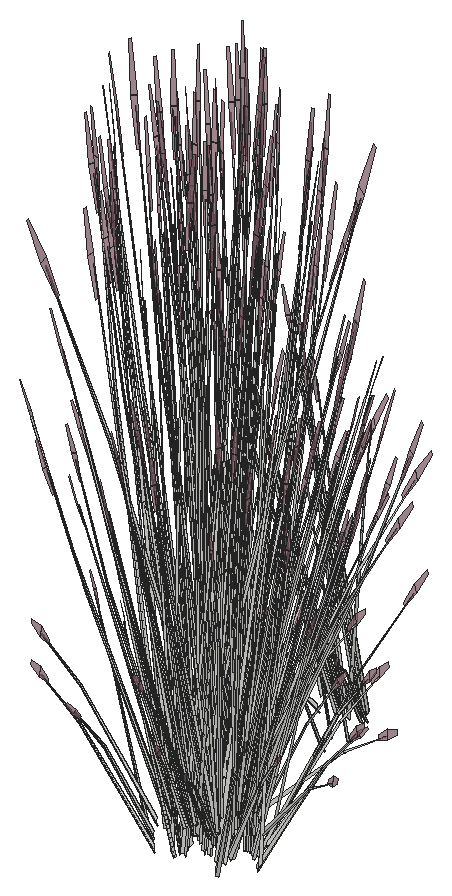
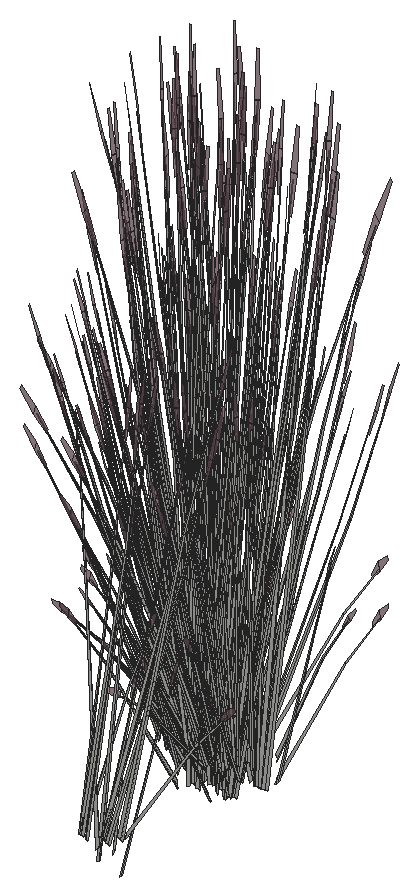
# SketchUp Ruby script. Lengths in inches.
U = 1.inch
M = Sketchup.active_model
def pt(a) = Geom::Point3d.new(a.map { |v| v * U })
def face(e, loops, mat)
  f = e.add_face(loops[0].map { |a| pt(a) })
  loops[1..].each { |l| e.add_face(l.map { |a| pt(a) }).erase! }
  f.material = f.back_material = mat if mat
  f
end
# faces: each face lists its corners as indices into pts; further lists are holes
def faces(e, pts, list, mat = nil) = list.each { |f| face(e, (f[0].is_a?(Array) ? f : [f]).map { |l| l.map { |i| pts[i] } }, mat) }
# xy, xz, yz: faces in a plane at the given z, y or x. An outline is a flat list of corners, or four numbers for a rectangle; further outlines are holes
def ring(l) = l.size == 4 ? [[l[0], l[1]], [l[2], l[1]], [l[2], l[3]], [l[0], l[3]]] : l.each_slice(2).to_a
def flat(e, list, mat, &to3) = list.each { |f| face(e, (f[0].is_a?(Array) ? f : [f]).map { |l| ring(l).map { |u, v| to3.(u, v) } }, mat) }
def xy(e, z, list, mat = nil) = flat(e, list, mat) { |x, y| [x, y, z] }
def xz(e, y, list, mat = nil) = flat(e, list, mat) { |x, z| [x, y, z] }
def yz(e, x, list, mat = nil) = flat(e, list, mat) { |y, z| [x, y, z] }
def lines(e, pts, list) = list.each { |a, b| e.add_line(pt(pts[a]), pt(pts[b])) }
# prism: a flat outline (further loops are holes) pulled along v
def prism(e, loops, v, mat = nil)
  f = face(e, loops, mat); d = Geom::Vector3d.new(v.map { |x| x * U })
  f.pushpull(f.normal.samedirection?(d) ? d.length : -d.length)
end
def box(e, o, s, mat = nil) = prism(e, [[o, [o[0] + s[0], o[1], o[2]], [o[0] + s[0], o[1] + s[1], o[2]], [o[0], o[1] + s[1], o[2]]]], [0, 0, s[2]], mat)
def at(x, y, z, deg = 0) = Geom::Transformation.translation(pt([x, y, z])) * Geom::Transformation.rotation(ORIGIN, Z_AXIS, deg.degrees)
def axes(o, x, y, z) = Geom::Transformation.new([*x, 0, *y, 0, *z, 0, *pt(o).to_a, 1])
def part(name) = M.definitions.add(name)
# library, detail: a bought-in or finely detailed component or shape, given as its bounding box
def library(name, o, s) = part(name).tap { |d| box(d.entities, o, s) }
def detail(e, o, s) = box(e.add_group.entities, o, s)
def put(e, d, t, mat = nil) = e.add_instance(d, t).tap { |i| i.material = mat if mat }
def group(e, t, mat = nil) = e.add_group.tap { |g| g.transformation = t; g.material = mat if mat }.entities
root = M.entities
M.materials.add("LightPink_Translucent").color = [144, 107, 117]
M.materials["LightPink_Translucent"].alpha = 0.75
c1 = part("blade")
p = [[2.15,0.21,22],[0,0.17,0],[0.09,0.45,0],[2.18,0.31,22],[2.29,0.31,22],[0.38,0.45,0],
  [2.48,0.24,33],[2.49,0.24,33],[2.48,0.22,33]]
faces(c1.entities,p,[[0,1,2,3],[4,5,2,3],[6,3,4,7],[8,0,3,6]])
c2 = part("seeds")
p = [[0.3,-0.1,1.38],[-0.01,-0.03,1.59],[-0.01,-0.03,0.03],[0.14,-0.07,-0.07],[0.29,-0.03,3],[0.15,0.01,3.11]]
faces(c2.entities,p,[[0,1,2,3],[1,0,4,5]],"LightPink_Translucent")
c3 = part("blade with seeds")
put(c3.entities,c1,at(0,0,0))
put(c3.entities,c2,axes([2.4,0.25,30.99],[1.5799,-0.05474,1.17369],[-0.12525,1.92788,0.29478],[-0.07173,-0.02425,1.56792]))
put(root,c3,axes([512.9,457.95,3.91],[-0.00733,-0.12161,1.74944],[-0.61946,-0.35147,-0.27667],[0.09577,-0.21306,0.14031]))
put(root,c3,axes([510.3,457.92,3.72],[0.22906,-0.4699,-0.35414],[0.66828,0.13705,0.4572],[-0.06128,-0.18919,0.87481]))
put(root,c3,axes([510.8,458.55,3.07],[-0.14147,0.21002,1.71376],[-0.59349,-0.43464,0.13857],[0.26773,-0.27089,0.73262]))
put(root,c3,axes([512.73,457.51,3.9],[-0.07716,0.04667,1.77383],[-0.75601,-0.15746,-0.16761],[-0.02737,-0.20368,0.31391]))
put(root,c3,axes([509.96,458.25,3.875],[-0.7469,-0.15318,-0.51099],[0.25601,-0.52518,-0.3958],[-0.06849,-0.21144,0.97773]))
put(root,c3,axes([510.42,456.93,1.96],[0.09747,0.35631,1.1486],[-0.54071,-0.19735,0.84392],[0.05818,-0.18244,0.25299]))
put(root,c3,axes([511.57,458.64,3.875],[-0.54391,-0.41056,-0.51099],[0.57458,-0.35956,-0.3958],[0.08276,-0.2086,0.97773]))
put(root,c3,axes([508.62,456.62,3.9],[-0.01417,0.07324,1.77383],[-0.6991,0.2658,-0.16761],[-0.20573,-0.13587,0.31391]))
put(root,c3,axes([508.46,457.92,4.29],[0.84639,-0.15705,0.53763],[0.14689,0.61608,0.4433],[-0.19906,-0.18157,1.11249]))
put(root,c3,axes([510.38,458.03,3.93],[0.74868,0.15974,0.48003],[-0.25601,0.52518,0.3958],[-0.04499,-0.20653,0.9933]))
put(root,c3,axes([510.59,458.22,4.23],[-0.74352,0.28449,-0.1216],[-0.36538,-0.50492,-0.67495],[-0.0981,-0.21277,1.02557]))
put(root,c3,axes([512.14,458.86,4.23],[-0.83505,-0.03027,-0.1216],[0.02282,-0.57322,-0.67495],[0.05801,-0.22077,1.02557]))
put(root,c3,axes([512.08,458.49,3.72],[0.5141,-0.32171,-0.35414],[0.48666,0.36734,0.4572],[0.07405,-0.18664,0.87481]))
put(root,c3,axes([507.64,457.36,1.96],[0.39634,0.21267,1.1486],[-0.57721,0.12784,0.84392],[-0.1235,-0.16344,0.25299]))
put(root,c3,axes([510.58,457.99,3.92],[0.55987,-0.20767,0.0643],[0.27403,0.37869,0.50621],[-0.05407,-0.16693,0.77189]))
put(root,c3,axes([508.37,458.1,3.72],[-0.11735,-0.49217,-0.35414],[0.67083,-0.12996,0.4572],[-0.18018,-0.14104,0.87481]))
put(root,c3,axes([508.66,458.05,3.92],[0.34533,-0.38816,0.0643],[0.49176,0.22599,0.50621],[-0.15898,-0.12445,0.77189]))
put(root,c3,axes([507.32,458,0.6875],[-0.0736,0.08049,1.76342],[-0.74378,0.17355,-0.26939],[-0.17968,-0.15788,0.30037]))
put(root,c3,axes([508.55,460.21,1.29],[-0.31203,-0.62659,-0.69835],[0.89884,-0.22566,-0.18329],[-0.03449,-0.21218,1.54149]))
put(root,c3,axes([512.72,458.3,0.6875],[-0.11372,-0.04814,1.76342],[-0.29211,-0.53779,-0.26939],[0.19706,-0.14594,0.30037]))
put(root,c3,axes([510.37,458.42,4.24],[-0.22906,0.4699,0.35414],[-0.66828,-0.13705,-0.4572],[-0.06128,-0.18919,0.87481]))
put(root,c3,axes([508.29,458.5,3.875],[-0.74975,0.14525,-0.51099],[-0.13115,-0.55007,-0.3958],[-0.20138,-0.15763,0.97773]))
put(root,c3,axes([512.08,458.62,3.93],[0.54105,0.41691,0.48003],[-0.57458,0.35956,0.3958],[0.0998,-0.1956,0.9933]))
put(root,c3,axes([512.28,458.66,3.92],[0.62439,0.02847,0.0643],[-0.01712,0.42991,0.50621],[0.06534,-0.16468,0.77189]))
put(root,c3,axes([511.8125,458.95,4.24],[-0.5141,0.32171,0.35414],[-0.48666,-0.36734,-0.4572],[0.07405,-0.18664,0.87481]))
put(root,c3,axes([512.72,459.8125,4.17],[0.39688,-0.48213,-0.71045],[0.69548,0.34264,0.08574],[0.23697,-0.17468,1.00501]))
put(root,c3,axes([508.43,458.41,1.57],[-0.47504,-0.61229,0],[0.79476,-0.34146,-0.51607],[0.18101,-0.07777,1.63711]))
put(root,c3,axes([512.7,459.59,3.875],[-0.19519,-0.55794,-0.51099],[0.73919,-0.0976,-0.3958],[0.21183,-0.14986,0.97773]))
put(root,c3,axes([509.47,457.67,1.32],[-0.52505,0.35054,-0.03893],[-0.48109,-0.38392,-0.17649],[-0.03387,-0.10878,0.58215]))
put(root,c3,axes([513.05,459.99,4.23],[-0.70283,-0.33692,-0.1216],[0.40491,-0.48793,-0.67495],[0.19857,-0.16961,1.02557]))
put(root,c3,axes([510.14,461.83,2.52],[0.65659,0.2464,1.51261],[-0.64324,0.53082,0.59816],[-0.28812,-0.31461,1.26806]))
put(root,c3,axes([508.77,458.5,4.24],[0.11735,0.49217,0.35414],[-0.67083,0.12996,-0.4572],[-0.18018,-0.14104,0.87481]))
put(root,c3,axes([506.71,460.125,1.21],[0,-0.61104,-0.49651],[0.85008,0,0],[0,-0.13917,1.57504]))
put(root,c3,axes([509.07,458.32,1.21],[0.7111,-0.30552,-0.49651],[0.42504,0.54784,0],[0.16196,-0.06958,1.57504]))
put(root,c3,axes([513.29,459.37,1.78],[-0.27143,-0.0181,1.43002],[-0.27808,-0.48551,-0.30754],[0.33346,-0.13735,0.61141]))
put(root,c3,axes([514.78,459.84,3.9],[-0.09924,-0.00464,1.77383],[-0.4121,-0.49725,-0.16761],[0.1655,-0.1635,0.31391]))
put(root,c3,axes([509.92,459.57,1.25],[0.51177,-0.45928,-0.62353],[0.63575,0.41646,-0.16365],[0.20507,-0.11457,1.37633]))
put(root,c3,axes([513.61,458.48,1.96],[-0.25308,0.31105,1.1486],[-0.21753,-0.4179,0.84392],[0.20902,-0.10472,0.25299]))
put(root,c3,axes([513.24,459.65,3.72],[0.66138,-0.08733,-0.35414],[0.17464,0.49921,0.4572],[0.18953,-0.13408,0.87481]))
put(root,c3,axes([509.02,460.375,1.4],[0.36864,-0.55059,-0.44739],[0.76598,0.26498,0.21531],[0,-0.12692,1.43643]))
put(root,c3,axes([509.36,460.1,1.86],[-0.08854,-0.69723,-0.29095],[0.92215,-0.04216,-0.50002],[0.16238,-0.09287,1.59708]))
put(root,c3,axes([507.08,460.14,1.22],[0.53038,-0.38124,-0.30978],[0.53038,0.38124,0.30978],[0,-0.1228,1.38974]))
put(root,c3,axes([506.86,458.31,1.32],[-0.21918,0.49894,-0.03893],[-0.6746,-0.15348,-0.17649],[-0.10242,-0.08161,0.58215]))
put(root,c3,axes([512.7,459.94,4.24],[-0.66138,0.08733,0.35414],[-0.17464,-0.49921,-0.4572],[0.18953,-0.13408,0.87481]))
put(root,c3,axes([508.93,460.83,1.86],[-0.85568,-0.29155,-0.29095],[0.41201,-0.61537,-0.50002],[-0.02689,-0.15109,1.59708]))
put(root,c3,axes([506.5,460.59,1.57],[-0.95008,0,0],[0,-0.68292,-0.51607],[0,-0.15554,1.63711]))
put(root,c3,axes([509.24,458.56,1.22],[0.70886,0.15119,-0.30978],[-0.17848,0.53243,0.30978],[0.1429,-0.0614,1.38974]))
put(root,c3,axes([513.3,459.86,3.92],[0.52161,0.25698,0.0643],[-0.30368,0.36595,0.50621],[0.16723,-0.11831,0.77189]))
put(root,c3,axes([513.16,459.76,3.93],[0.18844,0.56237,0.48003],[-0.73919,0.0976,0.3958],[0.21785,-0.13226,0.9933]))
put(root,c3,axes([515.15,460.4375,3.91],[0.10543,-0.09307,1.74944],[-0.13495,-0.57092,-0.27667],[0.26455,-0.10825,0.14031]))
put(root,c3,axes([507.23,460.41,1.52],[-0.70674,0.51372,0.30756],[-0.70717,-0.50832,-0.36492],[-0.02468,-0.14589,1.64885]))
put(root,c3,axes([509.48,460.65,1.625],[0.8561,0.29616,0.24065],[-0.41201,0.61537,0.50002],[0,-0.14185,1.60543]))
put(root,c3,axes([509.15,461.48,1.63],[0.20138,-0.72405,-0.23429],[0.95485,0.12621,0.51271],[-0.16685,-0.09999,1.5644]))
put(root,c3,axes([509.21,460.23,1.91],[-0.82508,0.03772,0.44739],[-0.07462,-0.62614,-0.21531],[0.14771,-0.06346,1.43643]))
put(root,c3,axes([507.08,460.69,1.67],[0,0.61104,0.49651],[-0.85008,0,0],[0,-0.13917,1.57504]))
put(root,c3,axes([513.08,461.3,4.23],[-0.38229,-0.5533,-0.1216],[0.6785,-0.2719,-0.67495],[0.28593,-0.073,1.02557]))
put(root,c3,axes([513.04,460.83,3.875],[0.20584,-0.55581,-0.51099],[0.70573,0.19051,-0.3958],[0.28414,-0.05097,0.97773]))
put(root,c3,axes([511.93,458.56,1.57],[0.47504,-0.61229,0],[0.79476,0.34146,-0.51607],[0.18101,0.07777,1.63711]))
put(root,c3,axes([509.08,461.18,1.4],[-0.45644,-0.51287,-0.44739],[0.69137,-0.36116,0.21531],[-0.14771,-0.06346,1.43643]))
put(root,c3,axes([509.18,460.46,1.55],[0.33034,0.68327,0.45755],[-0.94388,0.2376,0.17955],[0.01154,-0.12555,1.58856]))
put(root,c3,axes([513.8,460.98,1.17],[-0.48937,0.07333,1.41583],[-0.07789,-0.58369,0.08104],[0.34275,-0.08835,0.80566]))
put(root,c3,axes([514.6875,460.47,1.45],[-0.47106,-0.39072,-0.06488],[0.51591,-0.35801,-0.29416],[0.14618,-0.02521,0.97024]))
put(root,c3,axes([509.01,461,1.91],[-0.36864,0.55059,0.44739],[-0.76598,-0.26498,-0.21531],[0,-0.12692,1.43643]))
put(root,c3,axes([510.36,460.52,1.4],[0,-0.70701,0],[0.95008,0,0],[0,0,1.79456]))
put(root,c3,axes([511.52,458.88,1.67],[-0.7111,-0.30552,0.49651],[0.42504,-0.54784,0],[0.16196,0.06958,1.57504]))
put(root,c3,axes([512.91,461.03,4.17],[0.66765,-0.26986,-0.71045],[0.37208,0.55551,0.08574],[0.32259,-0.0631,1.00501]))
put(root,c3,axes([509.91,460.07,1.55],[-0.62999,0.55453,0.45755],[-0.74845,-0.4895,0.17955],[0.15188,-0.05534,1.58856]))
put(root,c3,axes([510.6,461.07,1.49],[-0.70674,-0.52593,-0.06131],[0.70717,-0.52625,0],[-0.02468,-0.01837,1.75571]))
put(root,c3,axes([508.82,459.16,1.67],[-0.21949,0.60727,0.17642],[-0.8032,-0.17185,0.35086],[0.13875,-0.00296,1.60407]))
put(root,c3,axes([512.81,461.14,4.24],[-0.63144,-0.17046,0.35414],[0.18417,-0.49731,-0.4572],[0.25423,-0.0456,0.87481]))
put(root,c3,axes([508.49,459.65,0.79],[-0.74787,0.24464,1.28929],[-0.23804,-0.70192,0.50096],[0.45924,0.01168,1.46642]))
put(root,c3,axes([510.5,459.83,1.81],[0.14658,-0.54532,0.1448],[0.71613,0.09466,-0.41347],[0.13033,0.05599,1.26744]))
put(root,c3,axes([509.26,461.13,1.55],[0.96033,0.12874,0.45755],[-0.19544,0.7271,0.17955],[-0.14034,-0.07021,1.58856]))
put(root,c3,axes([514.33,460.6,0.6875],[-0.03971,-0.09277,1.76342],[0.27541,-0.54264,-0.26939],[0.27782,-0.00781,0.30037]))
put(root,c3,axes([510.19,459.98,1.91],[-0.45644,-0.51287,0.44739],[0.69137,-0.36116,-0.21531],[0.14771,0.06346,1.43643]))
put(root,c3,axes([507.83,462.32,1.22],[-0.17848,-0.53243,-0.30978],[0.70886,-0.15119,0.30978],[-0.1429,-0.0614,1.38974]))
put(root,c3,axes([508.74,462.29,1.67],[0.81646,-0.16218,0.17642],[0.20161,0.60355,0.35086],[-0.07282,-0.08794,1.60407]))
put(root,c3,axes([510.43,460.01,1.86],[0.76714,-0.40567,-0.29095],[0.51013,0.57321,-0.50002],[0.18927,0.05821,1.59708]))
put(root,c3,axes([513.47,461.08,3.72],[0.63144,0.17046,-0.35414],[-0.18417,0.49731,0.4572],[0.25423,-0.0456,0.87481]))
put(root,c3,axes([507.64,462.55,1.21],[-0.7111,-0.30552,-0.49651],[0.42504,-0.54784,0],[-0.16196,-0.06958,1.57504]))
put(root,c3,axes([512.36,458.93,1.21],[0.7111,0.30552,-0.49651],[-0.42504,0.54784,0],[0.16196,0.06958,1.57504]))
put(root,c3,axes([511.01,460.68,1.4],[0.85008,0,0],[0,0.63259,0],[0,0,1.78407]))
put(root,c3,axes([509.57,461.47,1.86],[-0.76714,0.40567,-0.29095],[-0.51013,-0.57321,-0.50002],[-0.18927,-0.05821,1.59708]))
put(root,c3,axes([511.25,459.19,1.67],[-0.81646,0.16218,0.17642],[-0.20161,-0.60355,0.35086],[0.07282,0.08794,1.60407]))
put(root,c3,axes([511.75,460.47,3.07],[-0.31515,0.01384,1.71376],[0.20907,-0.5998,0.13857],[0.44912,0.0371,0.73262]))
put(root,c3,axes([512.16,459.16,1.22],[0.17848,0.53243,-0.30978],[-0.70886,0.15119,0.30978],[0.1429,0.0614,1.38974]))
put(root,c3,axes([513.38,461.29,3.92],[0.27906,0.41663,0.0643],[-0.50888,0.20393,0.50621],[0.22432,-0.04024,0.77189]))
put(root,c3,axes([510.73,460.35,1.57],[-0.96033,-0.12874,0.49198],[0.19544,-0.7271,0.19306],[0.14034,0.07021,1.70813]))
put(root,c3,axes([513.33,461.14,3.93],[-0.21466,0.55714,0.48003],[-0.70573,-0.19051,0.3958],[0.27753,-0.03348,0.9933]))
put(root,c3,axes([509.97,462.15,1.4],[-0.24791,-0.5268,0],[0.70791,-0.18448,0],[0,0,1.54371]))
put(root,c3,axes([509.5,461.65,1.81],[-0.14658,0.54532,0.1448],[-0.71613,-0.09466,-0.41347],[-0.13033,-0.05599,1.26744]))
put(root,c3,axes([510.9,462.08,1.38],[0.79769,-0.20732,-0.19198],[0.2803,0.59721,0.00008],[0.08805,-0.02292,1.73897]))
put(root,c3,axes([511.17,462.32,1.67],[0.21949,-0.60727,0.17642],[0.8032,0.17185,0.35086],[-0.13875,0.00296,1.60407]))
put(root,c3,axes([510.99,460.95,1.41],[0.53038,0.39469,0],[-0.53038,0.39469,0],[0,0,1.69266]))
put(root,c3,axes([512.43,460.78,1.67],[-0.59697,-0.44509,0.17642],[0.60159,-0.4317,0.35086],[-0.06593,0.0909,1.60407]))
put(root,c3,axes([511.32,460.1,1.25],[0.79037,0.10018,-0.62353],[-0.16679,0.61794,-0.16365],[0.23587,0.07488,1.37633]))
put(root,c3,axes([514.8125,461.18,1.96],[-0.46945,0.10088,1.1486],[0.22097,-0.4169,0.84392],[0.24904,0.02853,0.25299]))
put(root,c3,axes([509.79,462.39,1.39],[-0.76598,-0.27433,0],[0.36864,-0.57001,0],[0,0,1.62707]))
put(root,c3,axes([510.43,461.66,1.66],[-0.74193,-0.49181,-0.25192],[0.6243,-0.55226,0.5513],[-0.19979,0.05753,1.68216]))
put(root,c3,axes([508.48,462.6,1.67],[0.7111,0.30552,0.49651],[-0.42504,0.54784,0],[-0.16196,-0.06958,1.57504]))
put(root,c3,axes([510.98,460.49,1.91],[0.36864,-0.55059,0.44739],[0.76598,0.26498,-0.21531],[0,0.12692,1.43643]))
put(root,c3,axes([514.6,462.95,3.9],[-0.0687,-0.05349,1.77383],[0.15029,-0.57341,-0.16761],[0.27062,-0.03664,0.31391]))
put(root,c3,axes([510.84,460.8,1.48],[0,0.70667,-0.05637],[-0.95008,0,0],[0,0.02221,1.79368]))
put(root,c3,axes([510.91,460.3,1.4],[0.45644,0.51287,-0.44739],[-0.69137,0.36116,0.21531],[0.14771,0.06346,1.43643]))
put(root,c3,axes([514,462.47,3.12],[-0.14542,-0.51365,-0.03492],[0.68734,-0.11809,-0.15832],[0.14353,0.03256,0.52218]))
put(root,c3,axes([508.07,462.92,1.57],[-0.47504,0.61229,0],[-0.79476,-0.34146,-0.51607],[-0.18101,-0.07777,1.63711]))
put(root,c3,axes([512.22,462.45,4.23],[0.04068,-0.62141,-0.1216],[0.77029,0.01698,-0.67495],[0.29667,0.04317,1.02557]))
put(root,c3,axes([512.92,460.79,1.67],[0,-0.61104,0.49651],[0.85008,0,0],[0,0.13917,1.57504]))
put(root,c3,axes([510.79,461.25,1.91],[0.82508,-0.03772,0.44739],[0.07462,0.62614,-0.21531],[-0.14771,0.06346,1.43643]))
put(root,c3,axes([511.3,460.61,1.81],[0.70791,-0.1782,0.1448],[0.24791,0.50885,-0.41347],[0,0.11199,1.26744]))
put(root,c3,axes([512.1,462.21,4.24],[-0.43232,-0.38257,0.35414],[0.49364,-0.36215,-0.4572],[0.25081,0.0551,0.87481]))
put(root,c3,axes([510.05,461.55,1.4],[-0.82508,0.03772,-0.44739],[-0.07462,-0.62614,0.21531],[-0.14771,0.06346,1.43643]))
put(root,c3,axes([513.93,461.85,1.78],[-0.18299,-0.15028,1.43002],[0.23809,-0.49714,-0.30754],[0.37023,0.06735,0.61141]))
put(root,c3,axes([510.66,462.4,1.4],[0.76598,0.27433,0],[-0.36864,0.57001,0],[0,0,1.74954]))
put(root,c3,axes([512.89,462.08,3.91],[0.16299,-0.01033,1.74944],[0.44707,-0.47471,-0.27667],[0.28992,0.06266,0.14031]))
put(root,c3,axes([510.97,463.01,1.39],[-0.46912,-0.61443,-0.05142],[0.79476,-0.34146,0.51607],[-0.19584,0.0585,1.6363]))
put(root,c3,axes([510.8,461.52,1.81],[0.56134,0.36712,0.1448],[-0.46823,0.41419,-0.41347],[-0.13033,0.05599,1.26744]))
put(root,c3,axes([512.25,462.15,4.17],[0.75952,0.01471,-0.71045],[-0.05101,0.61953,0.08574],[0.32177,0.06538,1.00501]))
put(root,c3,axes([511.4,462.65,1.67],[0.7111,-0.30552,0.49651],[0.42504,0.54784,0],[-0.16196,0.06958,1.57504]))
put(root,c3,axes([510.39,462.17,1.48],[0.33034,0.70197,-0.06012],[-0.94388,0.24598,0],[0.01154,0.02451,1.72173]))
put(root,c3,axes([510.75,462.93,1.22],[-0.70886,-0.15119,-0.30978],[0.17848,-0.53243,0.30978],[-0.1429,0.0614,1.38974]))
put(root,c3,axes([506.82,461.43,4.24],[0.66138,-0.08733,0.35414],[0.17464,0.49921,-0.4572],[-0.18953,0.13408,0.87481]))
put(root,c3,axes([513.5,460.9,1.57],[0.95008,0,0],[0,0.68292,-0.51607],[0,0.15554,1.63711]))
put(root,c3,axes([513.12,461.25,1.39],[-0.94962,-0.00489,-0.04976],[0,-0.68292,0.49943],[-0.02984,0.15546,1.58352]))
put(root,c3,axes([511.0625,460.65,1.86],[0.85568,0.29155,-0.29095],[-0.41201,0.61537,-0.50002],[0.02689,0.15109,1.59708]))
put(root,c3,axes([512.71,462.41,3.72],[0.43232,0.38257,-0.35414],[-0.49364,0.36215,0.4572],[0.25081,0.0551,0.87481]))
put(root,c3,axes([512.92,461.35,1.22],[-0.53038,0.38124,-0.30978],[-0.53038,-0.38124,0.30978],[0,0.1228,1.38974]))
put(root,c3,axes([510.63,461.38,1.86],[0.08854,0.69723,-0.29095],[-0.92215,0.04216,-0.50002],[-0.16238,0.09287,1.59708]))
put(root,c3,axes([512.49,462.56,3.92],[-0.03826,0.46465,0.0643],[-0.57772,-0.01274,0.50621],[0.2213,0.04862,0.77189]))
put(root,c3,axes([510.97,461.11,1.4],[-0.36864,0.55059,-0.44739],[-0.76598,-0.26498,0.21531],[0,0.12692,1.43643]))
put(root,c3,axes([512.54,462.41,3.93],[-0.56024,0.40262,0.48003],[-0.48318,-0.42758,0.3958],[0.26285,0.07427,0.9933]))
put(root,c3,axes([505.32,462.85,4.84],[0.67048,0.16311,-0.06488],[-0.20625,0.50201,-0.29416],[-0.10966,0.07622,0.97024]))
put(root,c3,axes([510.08,461.92,1.25],[-0.51177,0.45928,-0.62353],[-0.63575,-0.41646,-0.16365],[-0.20507,0.11457,1.37633]))
put(root,c3,axes([510.76,462.875,4.24],[-0.11735,-0.49217,0.35414],[0.67083,-0.12996,-0.4572],[0.18018,0.14104,0.87481]))
put(root,c3,axes([510.99,462.69,1.52],[0.95122,0.19861,0.30756],[-0.23797,0.7099,-0.36492],[-0.15744,0.08885,1.64885]))
put(root,c3,axes([510.92,463.17,1.21],[-0.7111,0.30552,-0.49651],[-0.42504,-0.54784,0],[-0.16196,0.06958,1.57504]))
put(root,c3,axes([513.28,461.36,1.21],[0,0.61104,-0.49651],[-0.85008,0,0],[0,0.13917,1.57504]))
put(root,c3,axes([511.16,461.43,3.07],[-0.28223,-0.10528,1.71376],[0.58406,-0.44165,0.13857],[0.36402,0.19924,0.73262]))
put(root,c3,axes([511.21,460.04,3.67],[-0.65655,-0.31748,1.38283],[0.69326,-0.49431,0.59665],[0.21183,0.29789,1.33663]))
put(root,c3,axes([506.48,461.38,4.23],[0.70283,0.33692,-0.1216],[-0.40491,0.48793,-0.67495],[-0.19857,0.16961,1.02557]))
put(root,c3,axes([512.2,462.63,1.96],[-0.4278,-0.1757,1.1486],[0.5524,-0.17852,0.84392],[0.14899,0.15122,0.25299]))
put(root,c3,axes([510.7,463.13,4.23],[0.45276,-0.52302,-0.1216],[0.65568,0.30132,-0.67495],[0.22792,0.14777,1.02557]))
put(root,c3,axes([507.72,462.42,4.24],[0.5141,-0.32171,0.35414],[0.48666,0.36734,-0.4572],[-0.07405,0.18664,0.87481]))
put(root,c3,axes([511.57,463.07,1.57],[0.47504,0.61229,0],[-0.79476,0.34146,-0.51607],[-0.18101,0.07777,1.63711]))
put(root,c3,axes([510.11,463.5625,3.9],[0.00225,-0.07398,1.77383],[0.65113,-0.32638,-0.16761],[0.22617,0.1165,0.31391]))
put(root,c3,axes([512.32,463.28,0.6875],[0.05536,-0.08822,1.76342],[0.69692,-0.25981,-0.26939],[0.21129,0.13447,0.30037]))
put(root,c3,axes([511.16,460.65,2.03],[-0.02076,-0.57531,1.41272],[0.93937,0.14913,0.59816],[-0.22217,0.31481,1.3335]))
put(root,c3,axes([511.4,461.28,1.29],[0.2786,0.55945,-0.69212],[-0.80253,0.20149,-0.18165],[0.03079,0.18945,1.52773]))
put(root,c3,axes([507.25,462.71,3.92],[-0.62439,-0.02847,0.0643],[0.01712,-0.42991,0.50621],[-0.06534,0.16468,0.77189]))
put(root,c3,axes([507.45,462.75,3.93],[-0.54105,-0.41691,0.48003],[0.57458,-0.35956,0.3958],[-0.0998,0.1956,0.9933]))
put(root,c3,axes([511.24,462.87,3.875],[0.74975,-0.14525,-0.51099],[0.13115,0.55007,-0.3958],[0.20138,0.15763,0.97773]))
put(root,c3,axes([509.16,462.95,4.24],[0.22906,-0.4699,0.35414],[0.66828,0.13705,-0.4572],[0.06128,0.18919,0.87481]))
put(root,c3,axes([512.27,463.43,1.86],[-0.48723,-0.01916,1.0506],[0.32177,-0.40701,0.58006],[0.19248,0.1446,0.8241]))
put(root,c3,axes([510.87,463.32,3.92],[-0.34533,0.38816,0.0643],[-0.49176,-0.22599,0.50621],[0.15898,0.12445,0.77189]))
put(root,c3,axes([510.06,464.63,4.84],[0.52505,-0.35054,-0.06488],[0.48109,0.38392,-0.29416],[0.03387,0.10878,0.97024]))
put(root,c3,axes([511.01,463.21,3.93],[-0.75571,0.14023,0.48003],[-0.13115,-0.55007,0.3958],[0.17773,0.16212,0.9933]))
put(root,c3,axes([510.68,462.44,1.78],[0.01341,-0.20255,1.43002],[0.64074,-0.22625,-0.30754],[0.1978,0.24243,0.61141]))
put(root,c3,axes([508.95,463.38,3.92],[-0.55987,0.20767,0.0643],[-0.27403,-0.37869,0.50621],[0.05407,0.16693,0.77189]))
put(root,c3,axes([507.45,462.88,3.72],[-0.5141,0.32171,-0.35414],[-0.48666,-0.36734,0.4572],[-0.07405,0.18664,0.87481]))
put(root,c3,axes([507.39,462.51,4.59],[0.83505,0.03027,-0.13498],[-0.02282,0.57322,-0.74919],[-0.05801,0.22077,1.13838]))
put(root,c3,axes([508.93,463.15,4.23],[0.74352,-0.28449,-0.1216],[0.36538,0.50492,-0.67495],[0.0981,0.21277,1.02557]))
put(root,c3,axes([509.15,463.34,4.26],[-0.74868,-0.15974,0.53283],[0.25601,-0.52518,0.43934],[0.04499,0.20653,1.10256]))
put(root,c3,axes([507.77,464.13,1.96],[-0.01966,-0.36332,1.1486],[0.49135,0.25914,0.84392],[-0.09663,0.17317,0.25299]))
put(root,c3,axes([509.07,463.26,0.6875],[0.12297,-0.03325,1.76342],[0.73967,0.18301,-0.26939],[0.02163,0.20626,0.30037]))
put(root,c3,axes([507.96,462.73,4.2],[0.54391,0.41056,-0.5672],[-0.57458,0.35956,-0.43934],[-0.08276,0.2086,1.08528]))
put(root,c3,axes([507.37,463.34,2.02],[0.69024,-0.1082,0.06507],[0.15868,0.43593,-0.86304],[-0.04376,0.22067,0.7736]))
put(root,c3,axes([509.57,463.125,3.875],[0.7469,0.15318,-0.51099],[-0.25601,0.52518,-0.3958],[0.06849,0.21144,0.97773]))
put(root,c3,axes([510,462.04,3.07],[-0.17368,-0.19618,1.71376],[0.80256,-0.16516,0.13857],[0.18139,0.30799,0.73262]))
put(root,c3,axes([509.23,463.45,3.72],[-0.22906,0.4699,-0.35414],[-0.66828,-0.13705,0.4572],[0.06128,0.18919,0.87481]))
put(root,c3,axes([507.79,462.54,4.53],[-0.01977,0.56521,-0.7886],[-0.83252,-0.03796,0.09517],[-0.08786,0.23945,1.11556]))
put(root,c3,axes([505.61,464.02,3.9],[0.0862,-0.03689,1.77383],[0.71245,0.24539,-0.16761],[-0.01674,0.20431,0.31391]))
put(root,c3,axes([508.58,462.14,3.07],[-0.0186,-0.23452,1.71376],[0.80601,0.15558,0.13857],[-0.04985,0.33422,0.73262]))
put(root,c3,axes([509.3,463.03,4.17],[0.36264,0.49684,-0.71045],[-0.74649,0.27689,0.08574],[0.0848,0.24006,1.00501]))
put(root,c3,axes([507.2,463.81,1.78],[0.23977,-0.09639,1.43002],[0.59198,0.29065,-0.30754],[-0.1762,0.25149,0.61141]))
put(root,c3,axes([508.76,464.28,3.91],[0.09631,0.0984,1.74944],[0.77725,0.03866,-0.27667],[0.07816,0.217,0.14031]))
put(root,c3,axes([507.51,463.34,2.56],[0.01669,-0.31544,1.54345],[0.75083,0.16661,0.21329],[-0.06506,0.33618,0.72882]))
put(root,c3,axes([507.36,476.3,3.91],[-0.11621,-0.08567,1.74944],[-0.77555,0.05431,-0.27667],[-0.12378,-0.20491,0.14031]))
put(root,c3,axes([509.16,477.32,1.78],[-0.21597,0.12368,1.43002],[-0.64681,-0.21647,-0.30754],[0.1199,-0.26922,0.61141]))
put(root,c3,axes([508.17,477.75,4.17],[-0.36264,-0.49684,-0.71045],[0.74649,-0.27689,0.08574],[-0.0848,-0.24006,1.00501]))
put(root,c3,axes([507.55,476.65,0.6875],[-0.12744,0.02202,1.76342],[-0.70477,-0.24781,-0.26939],[0.01183,-0.2067,0.30037]))
put(root,c3,axes([509.68,478.23,4.17],[0.01977,-0.56521,-0.71045],[0.83252,0.03796,0.08574],[0.08786,-0.23945,1.00501]))
put(root,c3,axes([510.84,477.35,3.91],[-0.00733,-0.12161,1.74944],[-0.61946,-0.35147,-0.27667],[0.09577,-0.21306,0.14031]))
put(root,c3,axes([508.24,477.33,3.72],[0.22906,-0.4699,-0.35414],[0.66828,0.13705,0.4572],[-0.06128,-0.18919,0.87481]))
put(root,c3,axes([508.75,477.95,3.07],[-0.14147,0.21002,1.71376],[-0.59349,-0.43464,0.13857],[0.26773,-0.27089,0.73262]))
put(root,c3,axes([510.68,476.91,3.9],[-0.07716,0.04667,1.77383],[-0.75601,-0.15746,-0.16761],[-0.02737,-0.20368,0.31391]))
put(root,c3,axes([507.9,477.65,3.875],[-0.7469,-0.15318,-0.51099],[0.25601,-0.52518,-0.3958],[-0.06849,-0.21144,0.97773]))
put(root,c3,axes([508.36,476.33,1.96],[0.09747,0.35631,1.1486],[-0.54071,-0.19735,0.84392],[0.05818,-0.18244,0.25299]))
put(root,c3,axes([509.52,478.05,3.875],[-0.54391,-0.41056,-0.51099],[0.57458,-0.35956,-0.3958],[0.08276,-0.2086,0.97773]))
put(root,c3,axes([506.41,477.32,4.29],[0.84639,-0.15705,0.53763],[0.14689,0.61608,0.4433],[-0.19906,-0.18157,1.11249]))
put(root,c3,axes([508.33,477.43,3.93],[0.74868,0.15974,0.48003],[-0.25601,0.52518,0.3958],[-0.04499,-0.20653,0.9933]))
put(root,c3,axes([508.54,477.62,4.23],[-0.74352,0.28449,-0.1216],[-0.36538,-0.50492,-0.67495],[-0.0981,-0.21277,1.02557]))
put(root,c3,axes([510.09,478.26,4.23],[-0.83505,-0.03027,-0.1216],[0.02282,-0.57322,-0.67495],[0.05801,-0.22077,1.02557]))
